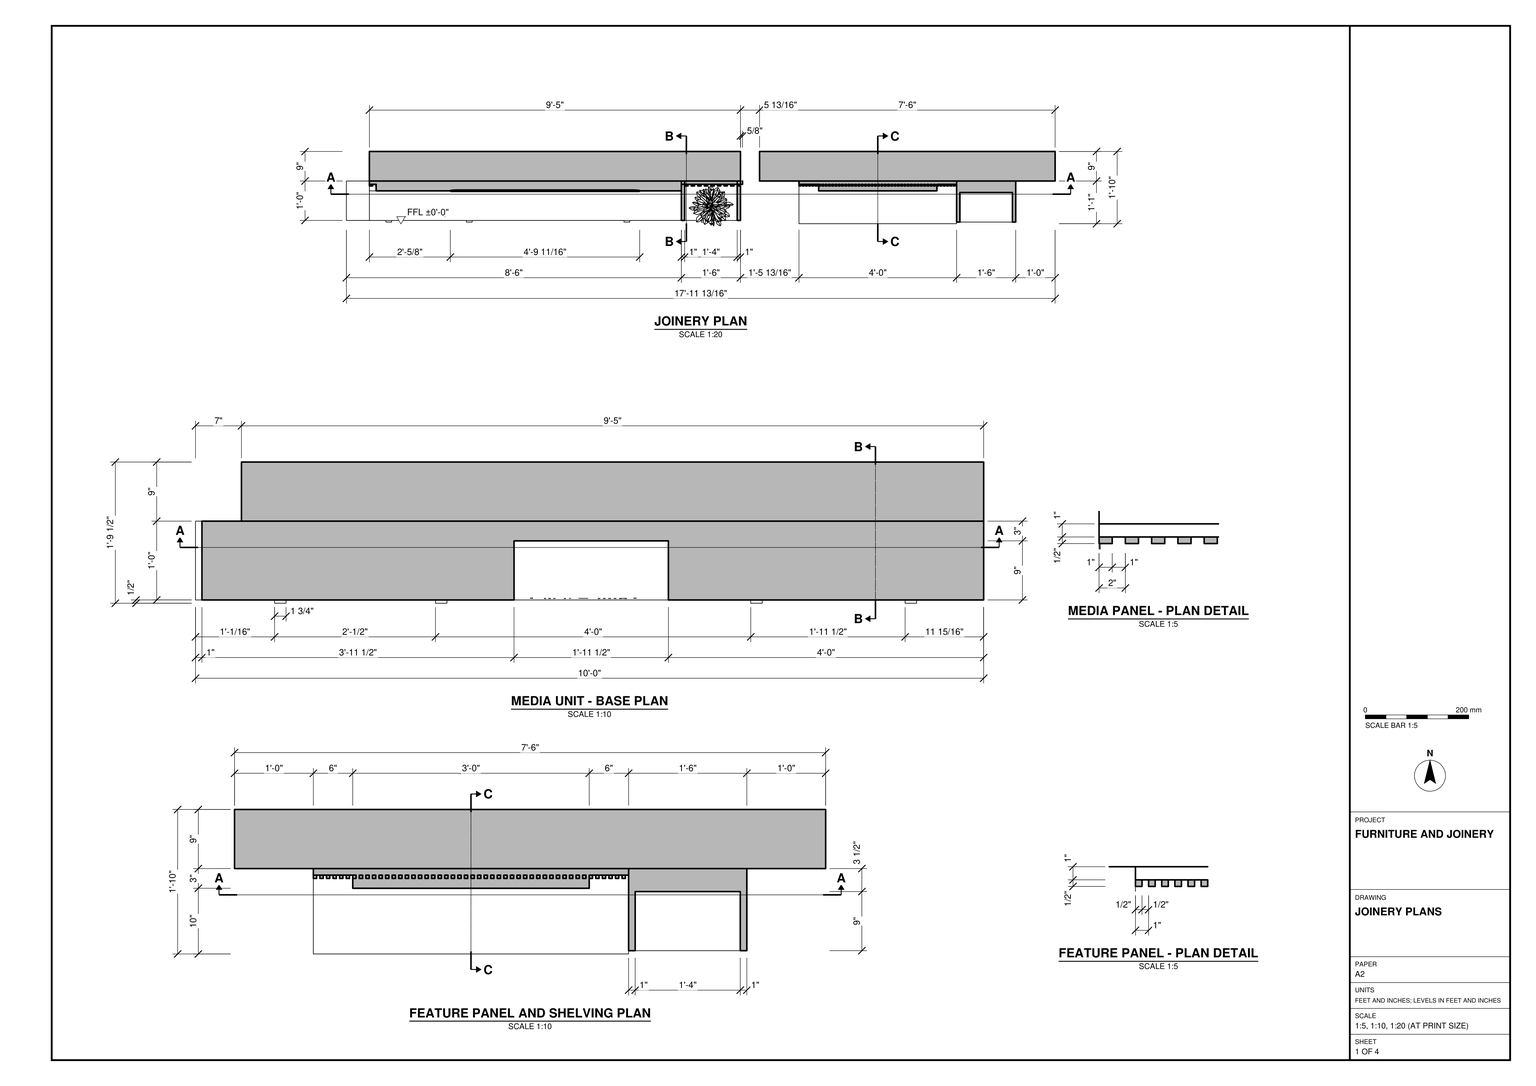
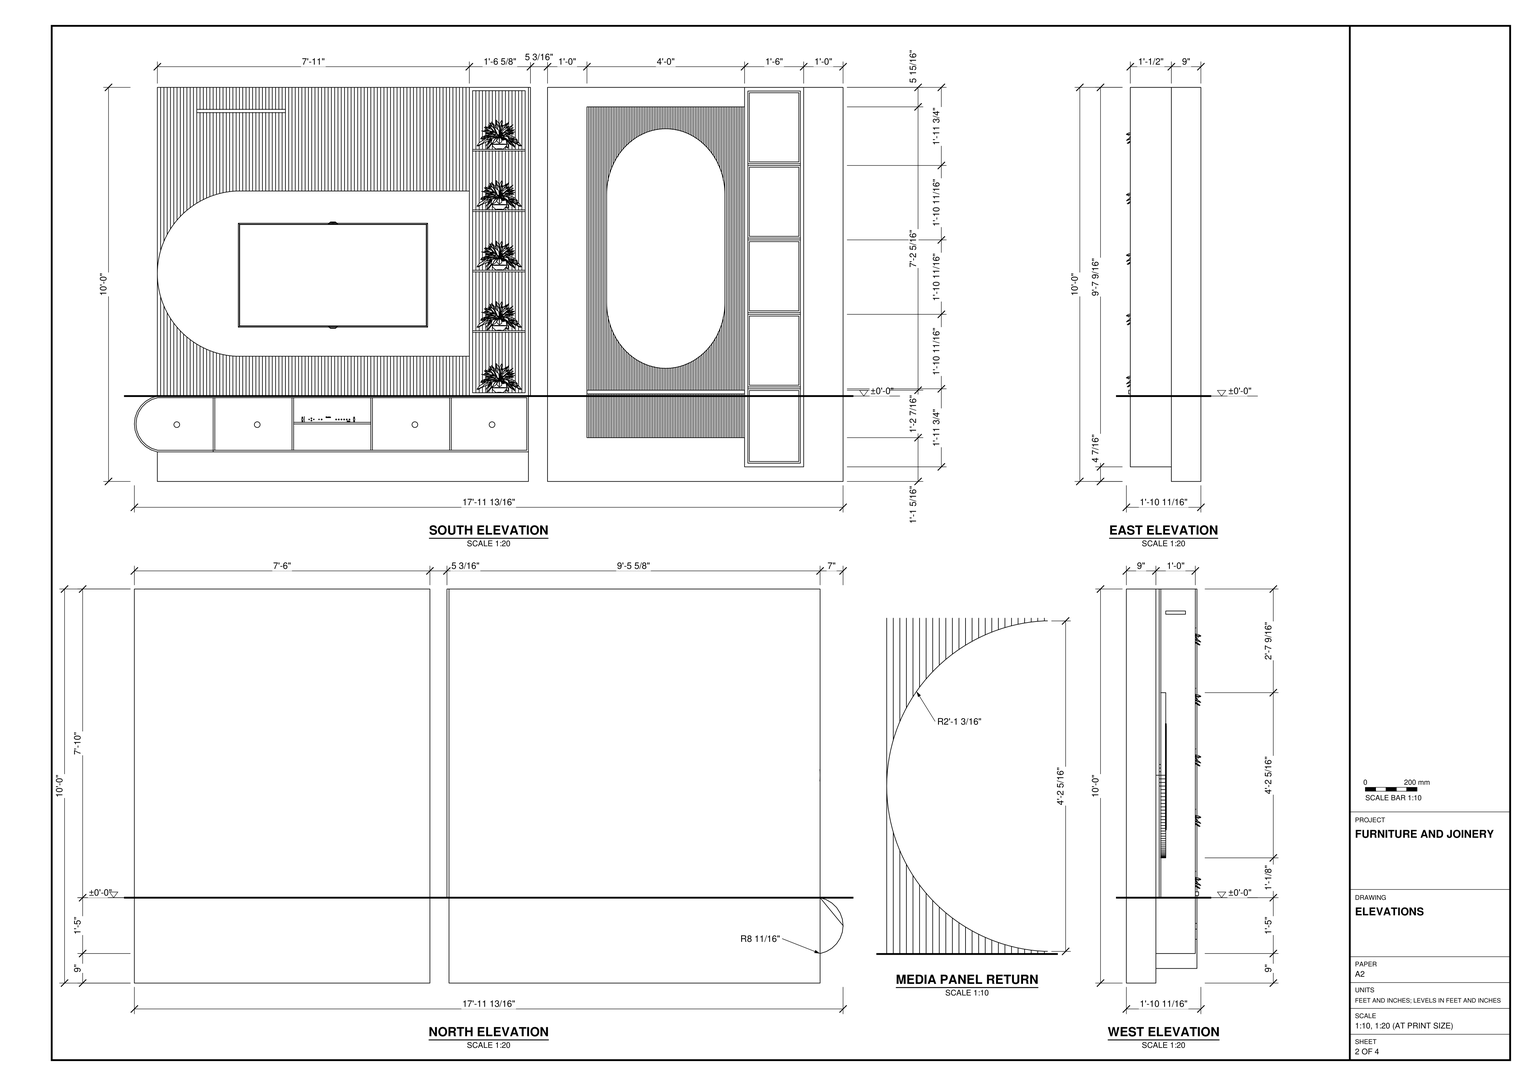
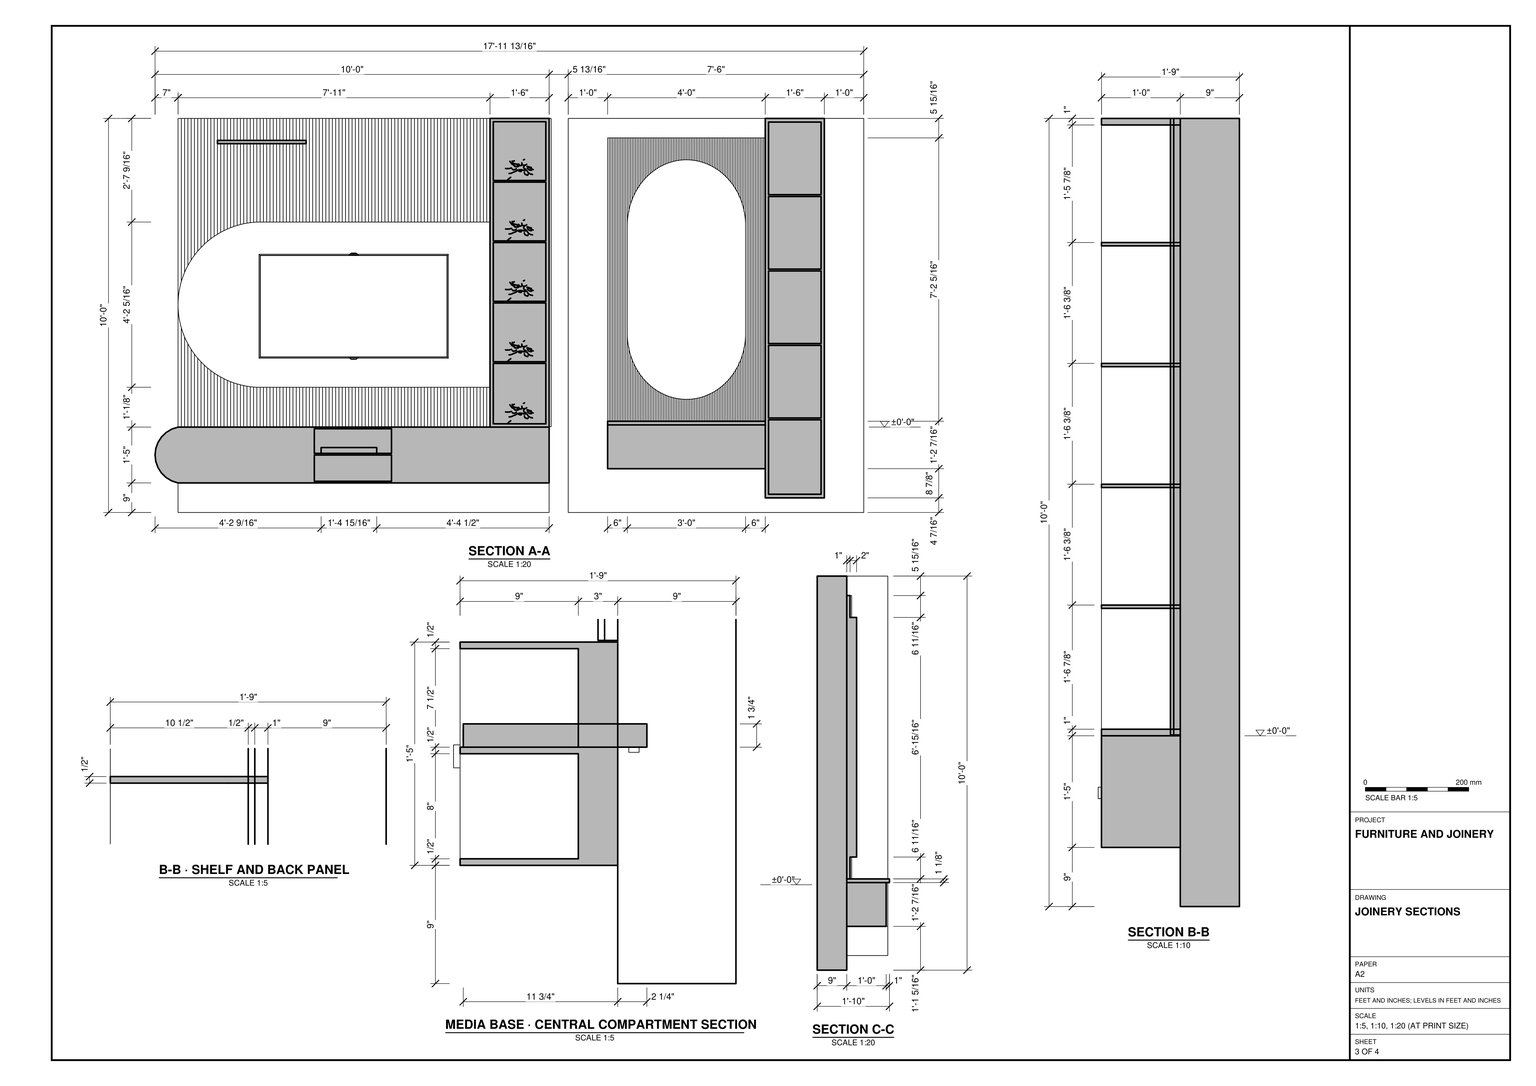
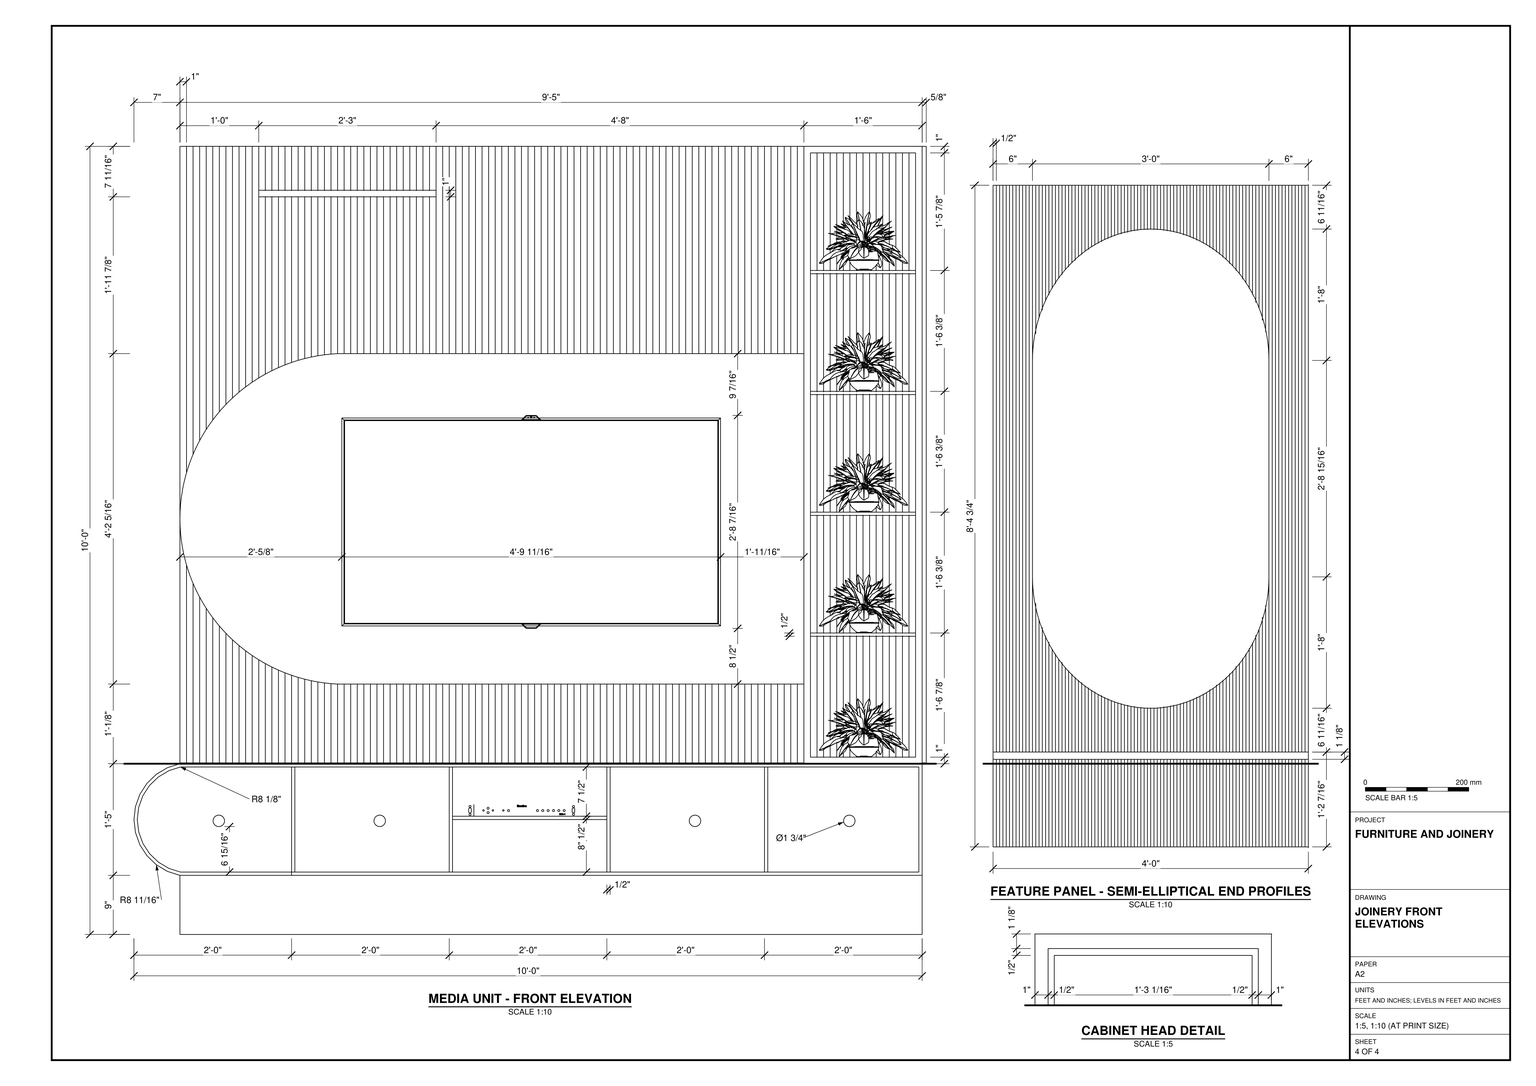
Build the joinery shown in task_files/diagram_01.pdf in SketchUp. Work in feet and inches. The complete assembly is 17'-11 13/16" wide, 1'-10 11/16" deep and 10'-0" high. Use the indicated ±0'-0" datum at the top of the media base. Extend the backing walls below this datum as shown in section.

Facing the joinery as in the south elevation, place the media unit on the left and the feature unit on the right, with a clear gap between their backing walls. Give the media base its rounded left end, divided cabinet fronts and recessed central equipment compartment. Above it, model the vertical slats around a horizontal screen panel with a semicircular left end. Finish the right edge of the media unit with a narrow column of display shelves.

On the companion unit, frame the upright capsule-shaped panel with finer vertical slats. Model the projecting base beneath it and the taller stack of open shelves immediately to its right. Follow the plans and sections for wall thicknesses, shelf depths and offsets between faces. Decor and loose items, including shelf plants and media equipment, may be any suitable library components. Keep the backing walls and each joinery or furniture piece in separate groups or components, and use components for repeated parts. Save one SketchUp model as output_files/media_wall_and_companion_feature_panel_with_shelving.skp.

# SketchUp Ruby script. Lengths in inches.
U = 1.inch
M = Sketchup.active_model
def pt(a) = Geom::Point3d.new(a.map { |v| v * U })
def face(e, loops, mat)
  f = e.add_face(loops[0].map { |a| pt(a) })
  loops[1..].each { |l| e.add_face(l.map { |a| pt(a) }).erase! }
  f.material = f.back_material = mat if mat
  f
end
# faces: each face lists its corners as indices into pts; further lists are holes
def faces(e, pts, list, mat = nil) = list.each { |f| face(e, (f[0].is_a?(Array) ? f : [f]).map { |l| l.map { |i| pts[i] } }, mat) }
# xy, xz, yz: faces in a plane at the given z, y or x. An outline is a flat list of corners, or four numbers for a rectangle; further outlines are holes
def ring(l) = l.size == 4 ? [[l[0], l[1]], [l[2], l[1]], [l[2], l[3]], [l[0], l[3]]] : l.each_slice(2).to_a
def flat(e, list, mat, &to3) = list.each { |f| face(e, (f[0].is_a?(Array) ? f : [f]).map { |l| ring(l).map { |u, v| to3.(u, v) } }, mat) }
def xy(e, z, list, mat = nil) = flat(e, list, mat) { |x, y| [x, y, z] }
def xz(e, y, list, mat = nil) = flat(e, list, mat) { |x, z| [x, y, z] }
def yz(e, x, list, mat = nil) = flat(e, list, mat) { |y, z| [x, y, z] }
def lines(e, pts, list) = list.each { |a, b| e.add_line(pt(pts[a]), pt(pts[b])) }
# prism: a flat outline (further loops are holes) pulled along v
def prism(e, loops, v, mat = nil)
  f = face(e, loops, mat); d = Geom::Vector3d.new(v.map { |x| x * U })
  f.pushpull(f.normal.samedirection?(d) ? d.length : -d.length)
end
def box(e, o, s, mat = nil) = prism(e, [[o, [o[0] + s[0], o[1], o[2]], [o[0] + s[0], o[1] + s[1], o[2]], [o[0], o[1] + s[1], o[2]]]], [0, 0, s[2]], mat)
def at(x, y, z, deg = 0) = Geom::Transformation.translation(pt([x, y, z])) * Geom::Transformation.rotation(ORIGIN, Z_AXIS, deg.degrees)
def axes(o, x, y, z) = Geom::Transformation.new([*x, 0, *y, 0, *z, 0, *pt(o).to_a, 1])
def part(name) = M.definitions.add(name)
# library, detail: a bought-in or finely detailed component or shape, given as its bounding box
def library(name, o, s) = part(name).tap { |d| box(d.entities, o, s) }
def detail(e, o, s) = box(e.add_group.entities, o, s)
def put(e, d, t, mat = nil) = e.add_instance(d, t).tap { |i| i.material = mat if mat }
def group(e, t, mat = nil) = e.add_group.tap { |g| g.transformation = t; g.material = mat if mat }.entities
root = M.entities
M.materials.add("[Basic Tile]").color = [203, 206, 202]
M.materials.add("[Color D01]").color = [255, 242, 204]
M.materials.add("[Color E01]").color = [255, 255, 204]
M.materials.add("[Color M00]").color = [255, 255, 255]
M.materials.add("[Color M07]").color = [58, 58, 58]
M.materials.add("[Mirror 01]").color = [185, 185, 185]
M.materials.add("[Wood Bamboo]").color = [177, 105, 43]
M.materials.add("[Wood Cherry Original]").color = [152, 86, 42]
c1 = library("Emotiva XDA-1",[0.14,0.2,-0.39],[16.93,14.02,2.16])
c2 = library("Television screen",[0,1.41,1.14],[35.92,0.28,20.21])
c3 = library("Group\#7",[0,0,0],[21.77,19.76,14.54])
c4 = part("Group\#3")
prism(c4.entities,[[[1.71,0,0.6],[1.75,0,0.83],[1.73,0,1.05],[1.65,0,1.27],[1.53,0,1.46],[1.35,0,1.61],[1.15,0,1.71],[0.92,0,1.75],[0.69,0,1.73],[0.48,0,1.65],[0.29,0,1.53],[0.14,0,1.35],[0.04,0,1.15],[0,0,0.92],[0.02,0,0.69],[0.09,0,0.48],[0.22,0,0.29],[0.39,0,0.14],[0.6,0,0.04],[0.83,0,0],[1.05,0,0.02],[1.27,0,0.09],[1.46,0,0.22],[1.61,0,0.39]]],[0,0.5,0])
c5 = library("Group50\#1",[-24,-6,0],[48,12,0.5])
c6 = library("Group101\#1",[-24,-38.83,0],[48,77.66,0.5])
c7 = library("Group135\#2",[-56.8125,-46.9375,0],[113,93.875,0.5])
put(root,c1,at(67.64,15.42,18,180))
g1 = group(root,at(0,-0.7,0),"[Wood Bamboo]")
put(g1,c2,axes([31.65,8.26,44.77],[1.605,0,0],[0,1.605,0],[0,0,1.605]))
put(g1,c3,axes([104.33,0,45.8],[0.62,0,0],[0,0.62,0],[0,0,0.62]))
put(g1,c3,axes([104.33,0,82.63],[0.62,0,0],[0,0.62,0],[0,0,0.62]))
put(g1,c3,axes([104.33,0,64.2],[0.62,0,0],[0,0.62,0],[0,0,0.62]))
put(g1,c3,axes([104.33,0,101.03],[0.62,0,0],[0,0.62,0],[0,0,0.62]))
g2 = group(g1,at(19,4.7,112.3125))
box(g2,[0,0,0],[27,6,1])
put(g1,c3,axes([104.33,0,26.9],[0.62,0,0],[0,0.62,0],[0,0,0.62]))
put(g1,c4,at(12.04,1.2,16.43),"[Color M07]")
put(g1,c4,at(36.54,1.2,16.43),"[Color M07]")
put(g1,c4,at(108.04,1.2,16.43),"[Color M07]")
put(g1,c4,at(84.54,1.2,16.43),"[Color M07]")
g3 = group(g1,at(0,1.7,9),"[Color M00]")
xy(g3,0,[[7,0,120,12]],"[Wood Bamboo]")
xy(g3,0.5,[[48.5,0,72,9]])
xy(g3,8.5,[[48.5,0,72,9]])
xy(g3,9,[[48.5,0,72,9]])
xy(g3,16.5,[[48.5,0,72,9]])
xy(g3,17,[[7,0,120,12]],"[Wood Bamboo]")
xz(g3,0,[[7,0,24,0,24,0.5,7.08,0.5,5.32,1.06,3.71,2.02,2.36,3.3125,1.35,4.88,0.72,6.64,0.5,8.5,0.72,10.36,1.35,12.12,2.36,13.6875,3.71,14.98,5.32,15.94,7.08,16.5,119.5,16.5,119.5,0.5,24,0.5,24,0,120,0,120,17,7,17,5.11,16.4,3.4,15.38,1.98,14.01,0.9,12.34,0.23,10.47,0,8.5,0.23,6.53,0.9,4.66,1.98,2.99,3.4,1.62,5.11,0.6],[7.08,0.5,24,0.5,24,16.5,7.08,16.5,5.32,15.94,3.71,14.98,2.36,13.6875,1.35,12.12,0.72,10.36,0.5,8.5,0.72,6.64,1.35,4.88,2.36,3.3125,3.71,2.02,5.32,1.06],[24,0.5,24.5,16.5],[24.5,0.5,48,16.5],[48,0.5,48.5,16.5],
  [72,0.5,72.5,16.5],[72.5,0.5,96,16.5],[96,0.5,96.5,16.5],[96.5,0.5,119.5,16.5],[48.5,8.5,72,9]])
xz(g3,9,[[48.5,0.5,72,8.5],[48.5,9,72,16.5]])
xz(g3,12,[[7,0,5.11,0.6,3.4,1.62,1.98,2.99,0.9,4.66,0.23,6.53,0,8.5,0.23,10.47,0.9,12.34,1.98,14.01,3.4,15.38,5.11,16.4,7,17,120,17,120,0]])
yz(g3,48.5,[[0,0.5,9,8.5],[0,9,9,16.5]])
yz(g3,72,[[0,0.5,9,8.5],[0,9,9,16.5]])
yz(g3,120,[[0,0,12,17]],"[Wood Bamboo]")
p = [[5.11,12,0.6],[7,12,0],[7,0,0],[5.11,0,0.6],[3.4,12,1.62],[3.4,0,1.62],
  [1.98,12,2.99],[1.98,0,2.99],[0.9,12,4.66],[0.9,0,4.66],[0.23,12,6.53],[0.23,0,6.53],
  [0,12,8.5],[0,0,8.5],[0.23,12,10.47],[0.23,0,10.47],[0.9,12,12.34],[0.9,0,12.34],
  [1.98,12,14.01],[1.98,0,14.01],[3.4,12,15.38],[3.4,0,15.38],[5.11,12,16.4],[5.11,0,16.4],
  [7,12,17],[7,0,17]]
faces(g3,p,[[0,1,2,3],[4,0,3,5],[6,4,5,7],[8,6,7,9],[10,8,9,11],[12,10,11,13],[14,12,13,15],[16,14,15,17],
  [18,16,17,19],[20,18,19,21],[22,20,21,23],[24,22,23,25]],"[Wood Bamboo]")
g4 = group(g1,at(0,13.7,0))
box(g4,[7,0,0],[113,9,120])
g5 = group(g1,at(102,1.7,26))
xy(g5,0,[[0,0,18,12]])
xy(g5,1,[[1,0,17,12]])
xy(g5,19.4,[[1,0,17,12]])
xy(g5,19.9,[[1,0,17,12]])
xy(g5,37.8,[[1,0,17,12]])
xy(g5,38.3,[[1,0,17,12]])
xy(g5,56.2,[[1,0,17,12]])
xy(g5,56.7,[[1,0,17,12]])
xy(g5,74.6,[[1,0,17,12]])
xy(g5,75.1,[[1,0,17,12]])
xy(g5,93,[[1,0,17,12]])
xy(g5,94,[[0,0,18,12]])
xz(g5,0,[[[0,0,18,94],[1,1,17,93]],[1,19.4,17,19.9],[1,37.8,17,38.3],[1,56.2,17,56.7],[1,74.6,17,75.1]])
xz(g5,12,[[[0,0,18,94],[1,1,17,19.4],[1,75.1,17,93],[1,56.7,17,74.6],[1,19.9,17,37.8],[1,38.3,17,56.2]]])
yz(g5,0,[[0,0,12,94]])
yz(g5,1,[[0,1,12,19.4],[0,19.9,12,37.8],[0,38.3,12,56.2],[0,56.7,12,74.6],[0,75.1,12,93]])
yz(g5,17,[[0,1,12,19.4],[0,19.9,12,37.8],[0,38.3,12,56.2],[0,56.7,12,74.6],[0,75.1,12,93]])
yz(g5,18,[[0,0,12,94]])
g6 = group(g1,at(7,10.7,26.125))
xy(g6,0,[[0,2,113.625,3]])
xy(g6,12,[[24,0,95,2]])
xy(g6,62.3125,[[24,0,95,2]])
xy(g6,93.875,[[0,2,113.625,3]])
xz(g6,0,[[24,12,95,12,95,62.3125,24,62.3125,22.91,62.24,21.82,62.11,20.73,61.94,19.66,61.73,18.6,61.46,17.54,61.15,16.51,60.8,15.49,60.4,14.48,59.95,13.5,59.47,12.54,58.9375,11.61,58.37,10.7,57.75,9.8125,57.1,8.96,56.42,8.14,55.69,7.35,54.93,6.59,54.14,5.87,53.3125,5.18,52.46,4.53,51.57,3.93,50.66,3.36,49.72,2.83,48.76,2.35,47.78,1.91,46.77,1.51,45.75,1.16,44.71,0.85,43.66,0.59,42.6,0.38,41.52,0.21,40.4375,0.1,39.35,0.02,38.25,0,37.16,0.02,36.06,0.1,34.97,0.21,33.875,0.38,32.79,0.59,31.72,0.85,30.65,1.16,29.6,1.51,28.5625,1.91,27.54,2.35,26.54,2.83,25.55,3.36,24.59,3.93,23.65,4.53,22.74,5.18,21.85,5.87,21,6.59,20.17,7.35,19.38,8.14,18.62,8.96,17.9,9.8125,17.21,10.7,16.56,11.61,15.95,12.54,15.375,13.5,14.85,14.48,14.36,15.49,13.91,16.51,13.51,17.54,13.16,18.6,12.85,19.66,12.59,20.73,12.37,21.82,12.2,22.91,12.08]],"[Basic Tile]")
xz(g6,2,[[0,0,113.625,0,113.625,93.875,0,93.875,0,37.16,0.02,38.25,0.1,39.35,0.21,40.4375,0.38,41.52,0.59,42.6,0.85,43.66,1.16,44.71,1.51,45.75,1.91,46.77,2.35,47.78,2.83,48.76,3.36,49.72,3.93,50.66,4.53,51.57,5.18,52.46,5.87,53.3125,6.59,54.14,7.35,54.93,8.14,55.69,8.96,56.42,9.8125,57.1,10.7,57.75,11.61,58.37,12.54,58.9375,13.5,59.47,14.48,59.95,15.49,60.4,16.51,60.8,17.54,61.15,18.6,61.46,19.66,61.73,20.73,61.94,21.82,62.11,22.91,62.24,24,62.3125,95,62.3125,95,12,24,12,22.91,12.08,21.82,12.2,20.73,12.37,19.66,12.59,18.6,12.85,17.54,13.16,16.51,13.51,15.49,13.91,14.48,14.36,13.5,14.85,12.54,15.375,11.61,15.95,10.7,16.56,9.8125,17.21,8.96,17.9,8.14,18.62,7.35,19.38,6.59,20.17,5.87,21,5.18,21.85,4.53,22.74,3.93,23.65,3.36,24.59,2.83,25.55,2.35,26.54,1.91,27.54,1.51,28.5625,1.16,29.6,0.85,30.65,0.59,31.72,0.38,32.79,0.21,33.875,0.1,34.97,0.02,36.06,0,37.16]])
yz(g6,0,[[2,0,3,37.16],[2,37.16,3,93.875]])
yz(g6,95,[[0,12,2,62.3125]])
yz(g6,113.625,[[2,0,3,93.875]])
p = [[22.91,2,12.08],[24,2,12],[24,0,12],[22.91,0,12.08],[21.82,2,12.2],[21.82,0,12.2],
  [20.73,2,12.37],[20.73,0,12.37],[19.66,2,12.59],[19.66,0,12.59],[18.6,2,12.85],[18.6,0,12.85],
  [17.54,2,13.16],[17.54,0,13.16],[16.51,2,13.51],[16.51,0,13.51],[15.49,2,13.91],[15.49,0,13.91],
  [14.48,2,14.36],[14.48,0,14.36],[13.5,2,14.85],[13.5,0,14.85],[12.54,2,15.375],[12.54,0,15.375],
  [11.61,2,15.95],[11.61,0,15.95],[10.7,2,16.56],[10.7,0,16.56],[9.8125,2,17.21],[9.8125,0,17.21],
  [8.96,2,17.9],[8.96,0,17.9],[8.14,2,18.62],[8.14,0,18.62],[7.35,2,19.38],[7.35,0,19.38],
  [6.59,2,20.17],[6.59,0,20.17],[5.87,2,21],[5.87,0,21],[5.18,2,21.85],[5.18,0,21.85],
  [4.53,2,22.74],[4.53,0,22.74],[3.93,2,23.65],[3.93,0,23.65],[3.36,2,24.59],[3.36,0,24.59],
  [2.83,2,25.55],[2.83,0,25.55],[2.35,2,26.54],[2.35,0,26.54],[1.91,2,27.54],[1.91,0,27.54],
  [1.51,2,28.5625],[1.51,0,28.5625],[1.16,2,29.6],[1.16,0,29.6],[0.85,2,30.65],[0.85,0,30.65],
  [0.59,2,31.72],[0.59,0,31.72],[0.38,2,32.79],[0.38,0,32.79],[0.21,2,33.875],[0.21,0,33.875],
  [0.1,2,34.97],[0.1,0,34.97],[0.02,2,36.06],[0.02,0,36.06],[0,2,37.16],[0,0,37.16],
  [0.02,2,38.25],[0.02,0,38.25],[0.1,2,39.35],[0.1,0,39.35],[0.21,2,40.4375],[0.21,0,40.4375],
  [0.38,2,41.52],[0.38,0,41.52],[0.59,2,42.6],[0.59,0,42.6],[0.85,2,43.66],[0.85,0,43.66],
  [1.16,2,44.71],[1.16,0,44.71],[1.51,2,45.75],[1.51,0,45.75],[1.91,2,46.77],[1.91,0,46.77],
  [2.35,2,47.78],[2.35,0,47.78],[2.83,2,48.76],[2.83,0,48.76],[3.36,2,49.72],[3.36,0,49.72],
  [3.93,2,50.66],[3.93,0,50.66],[4.53,2,51.57],[4.53,0,51.57],[5.18,2,52.46],[5.18,0,52.46],
  [5.87,2,53.3125],[5.87,0,53.3125],[6.59,2,54.14],[6.59,0,54.14],[7.35,2,54.93],[7.35,0,54.93],
  [8.14,2,55.69],[8.14,0,55.69],[8.96,2,56.42],[8.96,0,56.42],[9.8125,2,57.1],[9.8125,0,57.1],
  [10.7,2,57.75],[10.7,0,57.75],[11.61,2,58.37],[11.61,0,58.37],[12.54,2,58.9375],[12.54,0,58.9375],
  [13.5,2,59.47],[13.5,0,59.47],[14.48,2,59.95],[14.48,0,59.95],[15.49,2,60.4],[15.49,0,60.4],
  [16.51,2,60.8],[16.51,0,60.8],[17.54,2,61.15],[17.54,0,61.15],[18.6,2,61.46],[18.6,0,61.46],
  [19.66,2,61.73],[19.66,0,61.73],[20.73,2,61.94],[20.73,0,61.94],[21.82,2,62.11],[21.82,0,62.11],
  [22.91,2,62.24],[22.91,0,62.24],[24,2,62.3125],[24,0,62.3125]]
faces(g6,p,[[0,1,2,3],[4,0,3,5],[6,4,5,7],[8,6,7,9],[10,8,9,11],[12,10,11,13],[14,12,13,15],[16,14,15,17],
  [18,16,17,19],[20,18,19,21],[22,20,21,23],[24,22,23,25],[26,24,25,27],[28,26,27,29],[30,28,29,31],[32,30,31,33],
  [34,32,33,35],[36,34,35,37],[38,36,37,39],[40,38,39,41],[42,40,41,43],[44,42,43,45],[46,44,45,47],[48,46,47,49],
  [50,48,49,51],[52,50,51,53],[54,52,53,55],[56,54,55,57],[58,56,57,59],[60,58,59,61],[62,60,61,63],[64,62,63,65],
  [66,64,65,67],[68,66,67,69],[70,68,69,71],[72,70,71,73],[74,72,73,75],[76,74,75,77],[78,76,77,79],[80,78,79,81],
  [82,80,81,83],[84,82,83,85],[86,84,85,87],[88,86,87,89],[90,88,89,91],[92,90,91,93],[94,92,93,95],[96,94,95,97],
  [98,96,97,99],[100,98,99,101],[102,100,101,103],[104,102,103,105],[106,104,105,107],[108,106,107,109],[110,108,109,111],[112,110,111,113],
  [114,112,113,115],[116,114,115,117],[118,116,117,119],[120,118,119,121],[122,120,121,123],[124,122,123,125],[126,124,125,127],[128,126,127,129],
  [130,128,129,131],[132,130,131,133],[134,132,133,135],[136,134,135,137],[138,136,137,139],[140,138,139,141]])
g7 = group(root,at(125.8125,0,0))
g8 = group(g7,at(0,13,0),"[Color E01]")
box(g8,[0,0,0],[90,9,120])
g9 = group(g7,at(60,0.5,4.44))
xy(g9,0,[[0,0,18,12.5]],"[Wood Cherry Original]")
xy(g9,1.11,[[1,0,17,9]],"[Wood Cherry Original]")
xy(g9,23.78,[[1,0,17,9]],"[Wood Cherry Original]")
xy(g9,24.33,[[1,0,17,9]],"[Wood Cherry Original]")
xy(g9,46.44,[[1,0,17,9]],"[Wood Cherry Original]")
xy(g9,47,[[1,0,17,9]],"[Wood Cherry Original]")
xy(g9,69.11,[[1,0,17,9]],"[Wood Cherry Original]")
xy(g9,69.67,[[1,0,17,9]],"[Wood Cherry Original]")
xy(g9,91.78,[[1,0,17,9]],"[Wood Cherry Original]")
xy(g9,92.33,[[1,0,17,9]],"[Wood Cherry Original]")
xy(g9,114.44,[[1,0,17,9]],"[Wood Cherry Original]")
xy(g9,115.56,[[0,0,18,12.5]],"[Wood Cherry Original]")
xz(g9,0,[[[0,0,18,115.56],[1,1.11,17,114.44]],[1,23.78,17,24.33],[1,46.44,17,47],[1,69.11,17,69.67],[1,91.78,17,92.33]],"[Wood Cherry Original]")
xz(g9,9,[[[1,1.11,17,23.78],[1.47,1.63,16.53,23.26]],[[1,24.33,17,46.44],[1.47,24.86,16.53,45.92]],[[1,47,17,69.11],[1.47,47.52,16.53,68.59]],[[1,69.67,17,91.78],[1.47,70.1875,16.53,91.26]],[[1,92.33,17,114.44],[1.47,92.86,16.53,113.92]]],"[Color D01]")
xz(g9,9,[[1.47,1.63,16.53,23.26],[1.47,24.86,16.53,45.92],[1.47,47.52,16.53,68.59],[1.47,70.1875,16.53,91.26],[1.47,92.86,16.53,113.92]],"[Wood Cherry Original]")
xz(g9,12.5,[[0,0,18,115.56]],"[Wood Cherry Original]")
yz(g9,0,[[0,0,12.5,115.56]],"[Wood Cherry Original]")
yz(g9,1,[[0,1.11,9,23.78],[0,24.33,9,46.44],[0,47,9,69.11],[0,69.67,9,91.78],[0,92.33,9,114.44]],"[Wood Cherry Original]")
yz(g9,17,[[0,1.11,9,23.78],[0,24.33,9,46.44],[0,47,9,69.11],[0,69.67,9,91.78],[0,92.33,9,114.44]],"[Wood Cherry Original]")
yz(g9,18,[[0,0,12.5,115.56]],"[Wood Cherry Original]")
g10 = group(g7,at(12,1,13.33))
box(g10,[0,0,0],[48,12,13.33])
g11 = group(g10,at(0,-1,13.33))
box(g11,[0,0,0],[48,13,1.11])
put(g10,c5,axes([24,0,6.67],[1,0,0],[0,0,1.11111],[0,-1,0]),"[Wood Bamboo]")
g12 = group(g7,at(12,12,27.78))
xy(g12,0,[[0,0,48,1]])
xy(g12,86.3,[[0,0,48,1]])
xz(g12,-2,[[24,6.67,24.81,6.6875,25.61,6.75,26.42,6.85,27.21,6.99,28.01,7.17,28.79,7.39,29.5625,7.65,30.32,7.94,31.07,8.28,31.81,8.65,32.53,9.05,33.23,9.5,33.92,9.98,34.58,10.49,35.22,11.03,35.84,11.61,36.4375,12.21,37.01,12.85,37.56,13.51,38.07,14.2,38.5625,14.91,39.02,15.65,39.45,16.41,39.85,17.1875,40.22,17.99,40.55,18.81,40.85,19.64,41.12,20.49,41.35,21.35,41.55,22.22,41.71,23.1,41.84,23.98,41.93,24.875,41.98,25.77,42,26.67,42,59.63,41.98,60.53,41.93,61.42,41.84,62.3125,41.71,63.2,41.55,64.08,41.35,64.95,41.12,65.81,40.85,66.66,40.55,67.49,40.22,68.31,39.85,69.11,39.45,69.89,39.02,70.65,38.5625,71.38,38.07,72.1,37.56,72.79,37.01,73.45,36.4375,74.08,35.84,74.69,35.22,75.27,34.58,75.81,33.92,76.32,33.23,76.8,32.53,77.24,31.81,77.65,31.07,78.02,30.32,78.35,29.5625,78.65,28.79,78.91,28.01,79.13,27.21,79.31,26.42,79.45,25.61,79.55,24.81,79.61,24,79.63,23.19,79.61,22.39,79.55,21.58,79.45,20.79,79.31,19.99,79.13,19.21,78.91,18.4375,78.65,17.68,78.35,16.93,78.02,16.19,77.65,15.47,77.24,14.77,76.8,14.08,76.32,13.42,75.81,12.78,75.27,12.16,74.69,11.5625,74.08,10.99,73.45,10.44,72.79,9.93,72.1,9.4375,71.38,8.98,70.65,8.55,69.89,8.15,69.11,7.78,68.31,7.45,67.49,7.15,66.66,6.88,65.81,6.65,64.95,6.45,64.08,6.29,63.2,6.16,62.3125,6.07,61.42,6.02,60.53,6,59.63,6,26.67,6.02,25.77,6.07,24.875,6.16,23.98,6.29,23.1,6.45,22.22,6.65,21.35,6.88,20.49,7.15,19.64,7.45,18.81,7.78,17.99,8.15,17.1875,8.55,16.41,8.98,15.65,9.4375,14.91,9.93,14.2,10.44,13.51,10.99,12.85,11.5625,12.21,12.16,11.61,12.78,11.03,13.42,10.49,14.08,9.98,14.77,9.5,15.47,9.05,16.19,8.65,16.93,8.28,17.68,7.94,18.4375,7.65,19.21,7.39,19.99,7.17,20.79,6.99,21.58,6.85,22.39,6.75,23.19,6.6875]],"[Mirror 01]")
xz(g12,0,[[[0,0,48,86.3],[24,6.67,23.19,6.6875,22.39,6.75,21.58,6.85,20.79,6.99,19.99,7.17,19.21,7.39,18.4375,7.65,17.68,7.94,16.93,8.28,16.19,8.65,15.47,9.05,14.77,9.5,14.08,9.98,13.42,10.49,12.78,11.03,12.16,11.61,11.5625,12.21,10.99,12.85,10.44,13.51,9.93,14.2,9.4375,14.91,8.98,15.65,8.55,16.41,8.15,17.1875,7.78,17.99,7.45,18.81,7.15,19.64,6.88,20.49,6.65,21.35,6.45,22.22,6.29,23.1,6.16,23.98,6.07,24.875,6.02,25.77,6,26.67,6,59.63,6.02,60.53,6.07,61.42,6.16,62.3125,6.29,63.2,6.45,64.08,6.65,64.95,6.88,65.81,7.15,66.66,7.45,67.49,7.78,68.31,8.15,69.11,8.55,69.89,8.98,70.65,9.4375,71.38,9.93,72.1,10.44,72.79,10.99,73.45,11.5625,74.08,12.16,74.69,12.78,75.27,13.42,75.81,14.08,76.32,14.77,76.8,15.47,77.24,16.19,77.65,16.93,78.02,17.68,78.35,18.4375,78.65,19.21,78.91,19.99,79.13,20.79,79.31,21.58,79.45,22.39,79.55,23.19,79.61,24,79.63,24.81,79.61,25.61,79.55,26.42,79.45,27.21,79.31,28.01,79.13,28.79,78.91,29.5625,78.65,30.32,78.35,31.07,78.02,31.81,77.65,32.53,77.24,33.23,76.8,33.92,76.32,34.58,75.81,35.22,75.27,35.84,74.69,36.4375,74.08,37.01,73.45,37.56,72.79,38.07,72.1,38.5625,71.38,39.02,70.65,39.45,69.89,39.85,69.11,40.22,68.31,40.55,67.49,40.85,66.66,41.12,65.81,41.35,64.95,41.55,64.08,41.71,63.2,41.84,62.3125,41.93,61.42,41.98,60.53,42,59.63,42,26.67,41.98,25.77,41.93,24.875,41.84,23.98,41.71,23.1,41.55,22.22,41.35,21.35,41.12,20.49,40.85,19.64,40.55,18.81,40.22,17.99,39.85,17.1875,39.45,16.41,39.02,15.65,38.5625,14.91,38.07,14.2,37.56,13.51,37.01,12.85,36.4375,12.21,35.84,11.61,35.22,11.03,34.58,10.49,33.92,9.98,33.23,9.5,32.53,9.05,31.81,8.65,31.07,8.28,30.32,7.94,29.5625,7.65,28.79,7.39,28.01,7.17,27.21,6.99,26.42,6.85,25.61,6.75,24.81,6.6875]]])
xz(g12,1,[[0,0,48,86.3]])
yz(g12,0,[[0,0,1,86.3]])
yz(g12,6,[[-2,26.67,0,59.63]])
yz(g12,42,[[-2,26.67,0,59.63]])
yz(g12,48,[[0,0,1,86.3]])
p = [[21.58,0,6.85],[22.39,0,6.75],[22.39,-2,6.75],[21.58,-2,6.85],[23.19,0,6.6875],[23.19,-2,6.6875],
  [24,0,6.67],[24,-2,6.67],[24.81,0,6.6875],[24.81,-2,6.6875],[25.61,0,6.75],[25.61,-2,6.75],
  [26.42,0,6.85],[26.42,-2,6.85],[20.79,0,6.99],[20.79,-2,6.99],[27.21,0,6.99],[27.21,-2,6.99],
  [19.99,0,7.17],[19.99,-2,7.17],[28.01,0,7.17],[28.01,-2,7.17],[19.21,0,7.39],[19.21,-2,7.39],
  [28.79,0,7.39],[28.79,-2,7.39],[18.4375,0,7.65],[18.4375,-2,7.65],[29.5625,0,7.65],[29.5625,-2,7.65],
  [17.68,0,7.94],[17.68,-2,7.94],[30.32,0,7.94],[30.32,-2,7.94],[16.93,0,8.28],[16.93,-2,8.28],
  [31.07,0,8.28],[31.07,-2,8.28],[16.19,0,8.65],[16.19,-2,8.65],[31.81,0,8.65],[31.81,-2,8.65],
  [15.47,0,9.05],[15.47,-2,9.05],[32.53,0,9.05],[32.53,-2,9.05],[14.77,0,9.5],[14.77,-2,9.5],
  [33.23,0,9.5],[33.23,-2,9.5],[14.08,0,9.98],[14.08,-2,9.98],[33.92,0,9.98],[33.92,-2,9.98],
  [13.42,0,10.49],[13.42,-2,10.49],[34.58,0,10.49],[34.58,-2,10.49],[12.78,0,11.03],[12.78,-2,11.03],
  [35.22,0,11.03],[35.22,-2,11.03],[12.16,0,11.61],[12.16,-2,11.61],[35.84,0,11.61],[35.84,-2,11.61],
  [11.5625,0,12.21],[11.5625,-2,12.21],[36.4375,0,12.21],[36.4375,-2,12.21],[10.99,0,12.85],[10.99,-2,12.85],
  [37.01,0,12.85],[37.01,-2,12.85],[10.44,0,13.51],[10.44,-2,13.51],[37.56,0,13.51],[37.56,-2,13.51],
  [9.93,0,14.2],[9.93,-2,14.2],[38.07,0,14.2],[38.07,-2,14.2],[9.4375,0,14.91],[9.4375,-2,14.91],
  [38.5625,0,14.91],[38.5625,-2,14.91],[8.98,0,15.65],[8.98,-2,15.65],[39.02,0,15.65],[39.02,-2,15.65],
  [8.55,0,16.41],[8.55,-2,16.41],[39.45,0,16.41],[39.45,-2,16.41],[8.15,0,17.1875],[8.15,-2,17.1875],
  [39.85,0,17.1875],[39.85,-2,17.1875],[7.78,0,17.99],[7.78,-2,17.99],[40.22,0,17.99],[40.22,-2,17.99],
  [7.45,0,18.81],[7.45,-2,18.81],[40.55,0,18.81],[40.55,-2,18.81],[7.15,0,19.64],[7.15,-2,19.64],
  [40.85,0,19.64],[40.85,-2,19.64],[6.88,0,20.49],[6.88,-2,20.49],[41.12,0,20.49],[41.12,-2,20.49],
  [6.65,0,21.35],[6.65,-2,21.35],[41.35,0,21.35],[41.35,-2,21.35],[6.45,0,22.22],[6.45,-2,22.22],
  [41.55,0,22.22],[41.55,-2,22.22],[6.29,0,23.1],[6.29,-2,23.1],[41.71,0,23.1],[41.71,-2,23.1],
  [6.16,0,23.98],[6.16,-2,23.98],[41.84,0,23.98],[41.84,-2,23.98],[6.07,0,24.875],[6.07,-2,24.875],
  [41.93,0,24.875],[41.93,-2,24.875],[6.02,0,25.77],[6.02,-2,25.77],[41.98,0,25.77],[41.98,-2,25.77],
  [6,0,26.67],[6,-2,26.67],[42,0,26.67],[42,-2,26.67],[6.02,0,60.53],[6,0,59.63],
  [6,-2,59.63],[6.02,-2,60.53],[42,0,59.63],[41.98,0,60.53],[41.98,-2,60.53],[42,-2,59.63],
  [6.07,0,61.42],[6.07,-2,61.42],[41.93,0,61.42],[41.93,-2,61.42],[6.16,0,62.3125],[6.16,-2,62.3125],
  [41.84,0,62.3125],[41.84,-2,62.3125],[6.29,0,63.2],[6.29,-2,63.2],[41.71,0,63.2],[41.71,-2,63.2],
  [6.45,0,64.08],[6.45,-2,64.08],[41.55,0,64.08],[41.55,-2,64.08],[6.65,0,64.95],[6.65,-2,64.95],
  [41.35,0,64.95],[41.35,-2,64.95],[6.88,0,65.81],[6.88,-2,65.81],[41.12,0,65.81],[41.12,-2,65.81],
  [7.15,0,66.66],[7.15,-2,66.66],[40.85,0,66.66],[40.85,-2,66.66],[7.45,0,67.49],[7.45,-2,67.49],
  [40.55,0,67.49],[40.55,-2,67.49],[7.78,0,68.31],[7.78,-2,68.31],[40.22,0,68.31],[40.22,-2,68.31],
  [8.15,0,69.11],[8.15,-2,69.11],[39.85,0,69.11],[39.85,-2,69.11],[8.55,0,69.89],[8.55,-2,69.89],
  [39.45,0,69.89],[39.45,-2,69.89],[8.98,0,70.65],[8.98,-2,70.65],[39.02,0,70.65],[39.02,-2,70.65],
  [9.4375,0,71.38],[9.4375,-2,71.38],[38.5625,0,71.38],[38.5625,-2,71.38],[9.93,0,72.1],[9.93,-2,72.1],
  [38.07,0,72.1],[38.07,-2,72.1],[10.44,0,72.79],[10.44,-2,72.79],[37.56,0,72.79],[37.56,-2,72.79],
  [10.99,0,73.45],[10.99,-2,73.45],[37.01,0,73.45],[37.01,-2,73.45],[11.5625,0,74.08],[11.5625,-2,74.08],
  [36.4375,0,74.08],[36.4375,-2,74.08],[12.16,0,74.69],[12.16,-2,74.69],[35.84,0,74.69],[35.84,-2,74.69],
  [12.78,0,75.27],[12.78,-2,75.27],[35.22,0,75.27],[35.22,-2,75.27],[13.42,0,75.81],[13.42,-2,75.81],
  [34.58,0,75.81],[34.58,-2,75.81],[14.08,0,76.32],[14.08,-2,76.32],[33.92,0,76.32],[33.92,-2,76.32],
  [14.77,0,76.8],[14.77,-2,76.8],[33.23,0,76.8],[33.23,-2,76.8],[15.47,0,77.24],[15.47,-2,77.24],
  [32.53,0,77.24],[32.53,-2,77.24],[16.19,0,77.65],[16.19,-2,77.65],[31.81,0,77.65],[31.81,-2,77.65],
  [16.93,0,78.02],[16.93,-2,78.02],[31.07,0,78.02],[31.07,-2,78.02],[17.68,0,78.35],[17.68,-2,78.35],
  [30.32,0,78.35],[30.32,-2,78.35],[18.4375,0,78.65],[18.4375,-2,78.65],[29.5625,0,78.65],[29.5625,-2,78.65],
  [19.21,0,78.91],[19.21,-2,78.91],[28.79,0,78.91],[28.79,-2,78.91],[19.99,0,79.13],[19.99,-2,79.13],
  [28.01,0,79.13],[28.01,-2,79.13],[20.79,0,79.31],[20.79,-2,79.31],[27.21,0,79.31],[27.21,-2,79.31],
  [21.58,0,79.45],[21.58,-2,79.45],[26.42,0,79.45],[26.42,-2,79.45],[22.39,0,79.55],[22.39,-2,79.55],
  [25.61,0,79.55],[25.61,-2,79.55],[23.19,0,79.61],[23.19,-2,79.61],[24.81,0,79.61],[24.81,-2,79.61],
  [24,0,79.63],[24,-2,79.63],[42,0,24.875]]
faces(g12,p,[[0,1,2,3],[1,4,5,2],[4,6,7,5],[6,8,9,7],[8,10,11,9],[10,12,13,11],[14,0,3,15],[12,16,17,13],
  [18,14,15,19],[16,20,21,17],[22,18,19,23],[20,24,25,21],[26,22,23,27],[24,28,29,25],[30,26,27,31],[28,32,33,29],
  [34,30,31,35],[32,36,37,33],[38,34,35,39],[36,40,41,37],[42,38,39,43],[40,44,45,41],[46,42,43,47],[44,48,49,45],
  [50,46,47,51],[48,52,53,49],[54,50,51,55],[52,56,57,53],[58,54,55,59],[56,60,61,57],[62,58,59,63],[60,64,65,61],
  [66,62,63,67],[64,68,69,65],[70,66,67,71],[68,72,73,69],[74,70,71,75],[72,76,77,73],[78,74,75,79],[76,80,81,77],
  [82,78,79,83],[80,84,85,81],[86,82,83,87],[84,88,89,85],[90,86,87,91],[88,92,93,89],[94,90,91,95],[92,96,97,93],
  [98,94,95,99],[96,100,101,97],[102,98,99,103],[100,104,105,101],[106,102,103,107],[104,108,109,105],[110,106,107,111],[108,112,113,109],
  [114,110,111,115],[112,116,117,113],[118,114,115,119],[116,120,121,117],[122,118,119,123],[120,124,125,121],[126,122,123,127],[124,128,129,125],
  [130,126,127,131],[128,132,133,129],[134,130,131,135],[132,136,137,133],[138,134,135,139],[136,140,141,137],[142,143,144,145],[146,147,148,149],
  [150,142,145,151],[147,152,153,148],[154,150,151,155],[152,156,157,153],[158,154,155,159],[156,160,161,157],[162,158,159,163],[160,164,165,161],
  [166,162,163,167],[164,168,169,165],[170,166,167,171],[168,172,173,169],[174,170,171,175],[172,176,177,173],[178,174,175,179],[176,180,181,177],
  [182,178,179,183],[180,184,185,181],[186,182,183,187],[184,188,189,185],[190,186,187,191],[188,192,193,189],[194,190,191,195],[192,196,197,193],
  [198,194,195,199],[196,200,201,197],[202,198,199,203],[200,204,205,201],[206,202,203,207],[204,208,209,205],[210,206,207,211],[208,212,213,209],
  [214,210,211,215],[212,216,217,213],[218,214,215,219],[216,220,221,217],[222,218,219,223],[220,224,225,221],[226,222,223,227],[224,228,229,225],
  [230,226,227,231],[228,232,233,229],[234,230,231,235],[232,236,237,233],[238,234,235,239],[236,240,241,237],[242,238,239,243],[240,244,245,241],
  [246,242,243,247],[244,248,249,245],[250,246,247,251],[248,252,253,249],[254,250,251,255],[252,256,257,253],[258,254,255,259],[256,260,261,257],
  [262,258,259,263],[260,264,265,261],[266,262,263,267],[264,268,269,265],[270,266,267,271],[268,272,273,269],[274,270,271,275],[272,276,277,273],
  [278,274,275,279],[276,280,281,277],[282,278,279,283],[280,282,283,281]])
lines(g12,p,[[140,284]])
put(g12,c6,axes([24,0,43.15],[1,0,0],[0,0,1.11111],[0,-1,0]),"[Wood Bamboo]")
put(root,c7,axes([63.8125,12,73.0625],[1,0,0],[0,0,1],[0,-1,0]))
